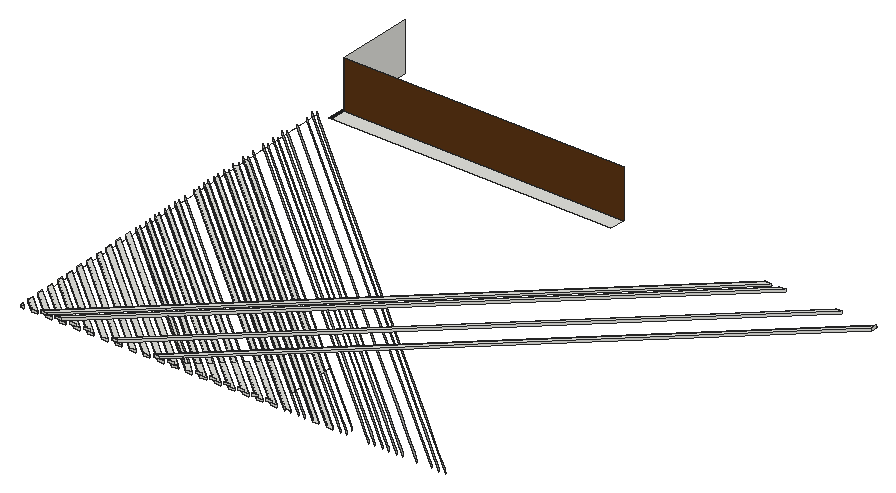
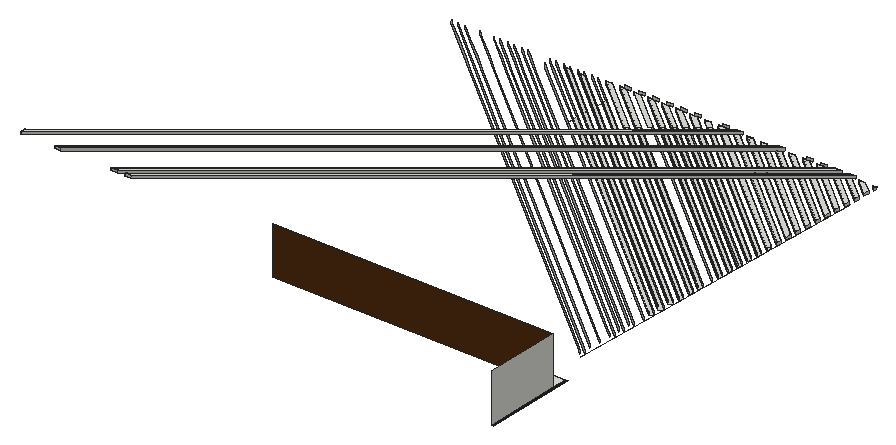
# SketchUp Ruby script. Lengths in inches.
U = 1.inch
M = Sketchup.active_model
def pt(a) = Geom::Point3d.new(a.map { |v| v * U })
def face(e, loops, mat)
  f = e.add_face(loops[0].map { |a| pt(a) })
  loops[1..].each { |l| e.add_face(l.map { |a| pt(a) }).erase! }
  f.material = f.back_material = mat if mat
  f
end
# faces: each face lists its corners as indices into pts; further lists are holes
def faces(e, pts, list, mat = nil) = list.each { |f| face(e, (f[0].is_a?(Array) ? f : [f]).map { |l| l.map { |i| pts[i] } }, mat) }
# xy, xz, yz: faces in a plane at the given z, y or x. An outline is a flat list of corners, or four numbers for a rectangle; further outlines are holes
def ring(l) = l.size == 4 ? [[l[0], l[1]], [l[2], l[1]], [l[2], l[3]], [l[0], l[3]]] : l.each_slice(2).to_a
def flat(e, list, mat, &to3) = list.each { |f| face(e, (f[0].is_a?(Array) ? f : [f]).map { |l| ring(l).map { |u, v| to3.(u, v) } }, mat) }
def xy(e, z, list, mat = nil) = flat(e, list, mat) { |x, y| [x, y, z] }
def xz(e, y, list, mat = nil) = flat(e, list, mat) { |x, z| [x, y, z] }
def yz(e, x, list, mat = nil) = flat(e, list, mat) { |y, z| [x, y, z] }
def lines(e, pts, list) = list.each { |a, b| e.add_line(pt(pts[a]), pt(pts[b])) }
# prism: a flat outline (further loops are holes) pulled along v
def prism(e, loops, v, mat = nil)
  f = face(e, loops, mat); d = Geom::Vector3d.new(v.map { |x| x * U })
  f.pushpull(f.normal.samedirection?(d) ? d.length : -d.length)
end
def box(e, o, s, mat = nil) = prism(e, [[o, [o[0] + s[0], o[1], o[2]], [o[0] + s[0], o[1] + s[1], o[2]], [o[0], o[1] + s[1], o[2]]]], [0, 0, s[2]], mat)
def at(x, y, z, deg = 0) = Geom::Transformation.translation(pt([x, y, z])) * Geom::Transformation.rotation(ORIGIN, Z_AXIS, deg.degrees)
def axes(o, x, y, z) = Geom::Transformation.new([*x, 0, *y, 0, *z, 0, *pt(o).to_a, 1])
def part(name) = M.definitions.add(name)
# library, detail: a bought-in or finely detailed component or shape, given as its bounding box
def library(name, o, s) = part(name).tap { |d| box(d.entities, o, s) }
def detail(e, o, s) = box(e.add_group.entities, o, s)
def put(e, d, t, mat = nil) = e.add_instance(d, t).tap { |i| i.material = mat if mat }
def group(e, t, mat = nil) = e.add_group.tap { |g| g.transformation = t; g.material = mat if mat }.entities
root = M.entities
M.materials.add("Wood066_2K_Color").color = [89, 51, 19]
M.materials.add("[Color M08]").color = [30, 30, 30]
xy(root,106.05,[[1644.4,661.04,1766.5625,667.76]])
xy(root,106.05,[[1643.34,661.04,1644.4,701.28]],"[Color M08]")
xz(root,667.76,[[1644.4,106.05,1766.5625,126.94]],"Wood066_2K_Color")
yz(root,1643.83,[[491.91,106.32,491.89,107.35,493.14,107.39,493.16,106.36],[496.17,106.47,498.52,106.55,498.5,107.58,496.15,107.5],[501.54,106.66,503.82,106.74,503.8,107.77,501.51,107.6875],[506.83,106.85,506.8125,107.875,509.17,107.96,509.1875,106.93],[512.2,107.04,512.18,108.06,514.47,108.15,514.49,107.12,512.95,107.0625],
  [517.5,107.23,517.48,108.25,519.83,108.34,519.85,107.31],[522.86,107.42,525.15,107.5,525.13,108.52,522.84,108.44],[528.16,107.6,530.51,107.6875,530.49,108.71,528.14,108.63],[533.53,107.79,535.74,107.87,535.72,108.9,533.5,108.82],[544.19,108.17,546.48,108.25,546.46,109.28,544.17,109.2]])
yz(root,1644.4,[[667.76,106.05,701.28,126.94]])
yz(root,1888.28,[[651.33,113.03,653.62,113.11,653.6,114.14,651.31,114.05]])
p = [[1673.29,491.89,107.35],[1643.83,517.48,108.25],[1643.83,517.5,107.23],[1673.29,491.91,106.32],[1643.83,519.85,107.31],[1676,491.91,106.32],
  [1676,491.89,107.35],[1643.83,519.83,108.34],[1643.83,512.2,107.04],[1643.83,512.95,107.0625],[1645.61,512.95,107.0625],[1669.83,491.91,106.32],
  [1667.19,491.91,106.32],[1643.83,514.49,107.12],[1643.83,514.47,108.15],[1669.83,491.89,107.35],[1667.19,491.89,107.35],[1643.83,512.18,108.06],
  [1643.83,493.16,106.36],[1645.27,491.91,106.32],[1643.83,491.91,106.32],[1645.27,491.89,107.35],[1643.83,491.89,107.35],[1643.83,493.14,107.39],
  [1643.83,496.17,106.47],[1643.83,496.15,107.5],[1648.74,491.89,107.35],[1648.74,491.91,106.32],[1643.83,498.52,106.55],[1651.45,491.91,106.32],
  [1651.45,491.89,107.35],[1643.83,498.5,107.58],[1691.74,491.91,106.32],[1643.83,533.53,107.79],[1643.83,535.74,107.87],[1643.87,535.78,107.875],
  [1694.38,491.91,106.32],[1691.74,491.89,107.35],[1643.83,533.5,108.82],[1679.47,491.91,106.32],[1643.83,522.86,107.42],[1643.83,525.15,107.5],
  [1682.1,491.91,106.32],[1679.47,491.89,107.35],[1643.83,522.84,108.44],[1682.1,491.89,107.35],[1643.83,525.13,108.52],[1697.84,491.91,106.32],
  [1643.83,538.83,107.98],[1643.83,541.18,108.07],[1700.55,491.91,106.32],[1700.55,491.89,107.35],[1643.81,541.19,108.07],[1643.81,541.17,109.09],
  [1643.83,541.16,109.09],[1697.84,491.89,107.35],[1643.83,538.8,109.01],[1710.12,491.89,107.35],[1643.83,549.47,109.39],[1643.83,549.49,108.36],
  [1710.12,491.91,106.32],[1643.83,551.84,108.44],[1712.83,491.91,106.32],[1712.83,491.89,107.35],[1643.83,551.82,109.47],[1711.88,492.72,107.375],
  [1716.3,491.91,106.32],[1643.83,554.85,108.55],[1643.83,557.14,108.63],[1718.93,491.91,106.32],[1713.61,494.22,107.43],[1643.83,554.83,109.58],
  [1716.3,491.89,107.35],[1714.93,495.37,107.47],[1718.93,491.89,107.35],[1643.83,557.12,109.66],[1722.4,491.91,106.32],[1643.83,560.15,108.74],
  [1643.83,562.51,108.82],[1725.11,491.91,106.32],[1716.66,496.87,107.52],[1643.83,560.13,109.76],[1722.4,491.89,107.35],[1718.02,498.05,107.5625],
  [1725.11,491.89,107.35],[1643.83,562.48,109.85],[1728.57,491.91,106.32],[1643.83,565.52,108.93],[1643.82,567.81,109.01],[1731.21,491.91,106.32],
  [1719.75,499.55,107.62],[1643.83,565.49,109.95],[1728.57,491.89,107.35],[1721.07,500.7,107.66],[1731.21,491.89,107.35],[1643.82,567.78,110.04],
  [1734.67,491.91,106.32],[1643.82,570.82,109.12],[1643.82,573.17,109.2],[1737.38,491.91,106.32],[1722.8,502.2,107.71],[1643.82,570.79,110.14],
  [1734.67,491.89,107.35],[1724.16,503.38,107.75],[1737.38,491.89,107.35],[1643.82,573.15,110.23],[1657.55,491.89,107.35],[1657.55,491.91,106.32],
  [1643.83,503.82,106.74],[1643.83,503.8,107.77],[1654.91,491.91,106.32],[1643.83,501.54,106.66],[1654.91,491.89,107.35],[1643.83,501.51,107.6875],
  [1740.85,491.91,106.32],[1643.82,576.18,109.31],[1643.82,578.47,109.39],[1743.49,491.92,106.32],[1725.89,504.89,107.81],[1643.82,576.16,110.33],
  [1740.85,491.89,107.35],[1727.21,506.03,107.85],[1743.49,491.89,107.35],[1643.82,578.45,110.41],[1663.72,491.89,107.35],[1663.72,491.91,106.32],
  [1643.83,509.1875,106.93],[1643.83,509.17,107.96],[1661.01,491.91,106.32],[1643.83,506.83,106.85],[1661.01,491.89,107.35],[1643.83,506.8125,107.875],
  [1753.93,501.88,106.67],[1765.4,491.92,106.32],[1765.4,491.89,107.35],[1738.16,515.55,108.18],[1643.82,597.48,111.09],[1643.82,597.51,110.0625],
  [1643.82,599.8,110.14],[1643.82,599.77,111.17],[1739.48,516.7,108.22],[1768.04,491.89,107.35],[1768.04,491.92,106.32],[1753.93,504.17,106.75],
  [1735.08,512.87,108.09],[1643.82,592.12,110.9],[1643.82,592.14,109.87],[1753.93,496.51,106.48],[1759.23,491.92,106.32],[1759.23,491.89,107.35],
  [1736.43,514.05,108.13],[1761.9375,491.89,107.35],[1761.9375,491.92,106.32],[1753.93,498.87,106.56],[1643.82,594.5,109.96],[1643.82,594.47,110.98],
  [1753.93,517.84,107.24],[1783.78,491.92,106.32],[1783.78,491.89,107.35],[1782.87,492.6875,107.375],[1781.3,494.05,107.42],[1778.04,496.88,107.52],
  [1747.35,523.53,108.47],[1643.82,613.45,111.65],[1643.82,613.47,110.63],[1728.9375,507.54,107.9],[1643.82,581.46,110.52],[1643.82,581.48,109.49],
  [1746.95,491.92,106.32],[1746.95,491.89,107.35],[1732.03,510.22,108],[1643.82,586.82,110.71],[1643.82,586.84,109.68],[1753.13,491.92,106.32],
  [1753.13,491.89,107.35],[1643.82,589.13,109.77],[1753.93,493.5,106.375],[1753.93,491.92,106.32],[1733.34,511.36,108.04],[1755.76,491.89,107.35],
  [1755.76,491.92,106.32],[1643.82,589.11,110.79],[1685.57,491.89,107.35],[1643.83,528.14,108.63],[1643.83,528.16,107.6],[1685.57,491.91,106.32],
  [1643.83,530.51,107.6875],[1688.28,491.91,106.32],[1688.28,491.89,107.35],[1643.83,530.49,108.71],[1753.93,507.18,106.86],[1643.82,602.81,110.25],
  [1645.18,603.98,110.29],[1774.21,491.92,106.32],[1771.5,491.92,106.32],[1771.5,491.89,107.35],[1741.21,518.2,108.28],[1643.82,602.78,111.28],
  [1753.93,512.54,107.05],[1753.93,512.95,107.0625],[1753.46,512.95,107.0625],[1643.82,608.17,110.44],[1645.14,609.32,110.48],[1780.32,491.92,106.32],
  [1777.68,491.92,106.32],[1777.68,491.89,107.35],[1774.99,494.23,107.43],[1744.3,520.88,108.375],[1643.82,608.15,111.47],[1704.02,491.91,106.32],
  [1643.83,544.19,108.17],[1643.83,546.48,108.25],[1706.66,491.91,106.32],[1643.83,546.46,109.28],[1706.66,491.89,107.35],[1704.02,491.89,107.35],
  [1643.83,544.17,109.2],[1753.93,528.5,107.62],[1796.06,491.92,106.32],[1796.06,491.9,107.35],[1792.05,495.375,107.47],[1784.18,502.22,107.71],
  [1753.49,528.87,108.66],[1643.82,624.11,112.03],[1643.82,624.13,111.01],[1753.93,533.87,107.81],[1802.23,491.92,106.32],[1802.23,491.9,107.35],
  [1795.14,498.06,107.5625],[1787.26,504.9,107.81],[1756.58,531.55,108.75],[1643.82,629.48,112.22],[1643.82,629.5,111.2],[1753.93,539.17,107.99],
  [1808.33,491.92,106.32],[1808.33,491.9,107.35],[1798.19,500.71,107.66],[1790.3125,507.55,107.9],[1759.625,534.2,108.85],[1643.82,634.77,112.41],
  [1643.82,634.8,111.38],[1753.93,555.2,108.5625],[1826.79,491.92,106.32],[1826.79,491.9,107.35],[1817.97,499.56,107.62],[1807.42,508.72,107.94],
  [1799.54,515.5625,108.18],[1768.85,542.21,109.13],[1647.16,647.9,112.875],[1643.82,650.8,112.98],[1643.82,650.82,111.95],[1694.38,491.89,107.35],
  [1643.87,535.76,108.9],[1776.3,495.38,107.47],[1780.32,491.89,107.35],[1645.14,609.29,111.51],[1645.82,608.7,111.49],[1745.62,522.03,108.41],
  [1797.77,498.06,107.5625],[1803.55,493.04,107.39],[1803.91,492.73,107.375],[1804.87,491.9,107.35],[1804.87,491.92,106.32],[1753.93,536.16,107.89],
  [1648.23,627.96,111.14],[1645.14,630.64,111.24],[1645.14,630.62,112.26],[1645.85,630,112.24],[1757.89,532.69,108.79],[1788.58,506.04,107.85],
  [1796.46,499.2,107.6],[1813.15,495.37,107.47],[1815.83,493.04,107.39],[1817.15,491.9,107.35],[1817.15,491.92,106.32],[1753.93,546.82,108.27],
  [1645.14,641.31,111.61],[1645.14,641.28,112.64],[1645.91,640.62,112.62],[1648.65,638.24,112.53],[1764.03,538.02,108.98],[1794.72,511.375,108.04],
  [1802.6,504.53,107.79],[1812.16,496.23,107.5],[1819.29,500.7,107.66],[1828.1,493.04,107.39],[1829.42,491.9,107.35],[1829.42,491.92,106.32],
  [1753.93,557.48,108.64],[1649.02,648.59,111.875],[1645.14,651.97,111.99],[1645.14,651.95,113.02],[1648.69,648.86,112.91],[1770.17,543.36,109.17],
  [1800.86,516.71,108.23],[1808.73,509.86,107.98],[1783.12,494.82,107.45],[1784.22,493.86,107.42],[1786.49,491.9,107.35],[1786.49,491.92,106.32],
  [1781.35,496.38,106.48],[1753.93,520.19,107.32],[1645.18,614.65,110.67],[1645.18,614.625,111.7],[1645.43,614.4,111.6875],[1748.71,524.71,108.51],
  [1779.39,498.06,107.5625],[1773.25,492.73,107.375],[1774.21,491.89,107.35],[1645.18,603.96,111.32],[1645.47,603.71,111.31],[1742.57,519.38,108.32],
  [1811.04,491.9,107.35],[1811.04,491.92,106.32],[1753.93,541.52,108.08],[1649.32,632.37,111.3],[1645.17,635.97,111.43],[1645.17,635.95,112.45],
  [1648.86,632.75,112.34],[1760.98,535.375,108.89],[1791.67,508.72,107.94],[1799.55,501.88,107.7],[1807.24,495.2,107.46],[1810.1,492.72,107.375],
  [1793.41,496.55,107.51],[1797.41,493.07,107.39],[1798.77,491.9,107.35],[1798.77,491.92,106.32],[1753.93,530.86,107.7],[1645.17,625.31,111.05],
  [1645.17,625.29,112.07],[1648.82,622.12,111.96],[1754.84,530.04,108.7],[1785.53,503.39,107.75],[1788.05,501.21,107.68],[1797.81,514.06,108.13],
  [1802.64,509.86,107.98],[1805.68,507.21,107.89],[1816.24,498.05,107.5625],[1823.32,491.9,107.35],[1823.32,491.92,106.32],[1753.93,552.18,108.46],
  [1649.5,642.88,111.67],[1645.17,646.64,111.8],[1645.17,646.61,112.83],[1648.5,643.72,112.73],[1767.12,540.71,109.08],[1655.64,491.89,107.35],
  [1661.81,491.89,107.35],[1667.91,491.89,107.35],[1674.09,491.89,107.35],[1686.36,491.89,107.35],[1704.74,491.89,107.35],[1712.46,491.89,107.35],
  [1710.93,491.89,107.35],[1723.19,491.89,107.35],[1729.3,491.89,107.35],[1735.47,491.89,107.35],[1741.57,491.89,107.35],[1749.66,491.89,107.35],
  [1749.66,491.92,106.32],[1747.75,491.89,107.35],[1753.85,491.89,107.35],[1784.75,496.44,106.48],[1785.96,495.39,106.44],[1785.96,495.37,107.47],
  [1782.86,498.06,107.5625],[1781.125,499.57,107.62],[1750.4375,526.22,108.5625],[1643.82,618.8125,111.85],[1643.82,618.83,110.82],[1753.93,523.21,107.43],
  [1643.83,535.72,108.9],[1653,491.89,107.375],[1653,491.89,107.35],[1655.64,491.89,107.375],[1655.64,491.86,108.4],[1653,491.86,108.4],
  [1659.1,491.86,108.4],[1659.1,491.89,107.375],[1659.1,491.89,107.35],[1661.81,491.89,107.375],[1661.81,491.86,108.4],[1665.28,491.89,107.35],
  [1667.91,491.89,107.375],[1667.91,491.86,108.4],[1665.28,491.86,108.4],[1665.28,491.89,107.375],[1671.38,491.89,107.35],[1674.09,491.89,107.375],
  [1674.09,491.87,108.4],[1671.38,491.86,108.4],[1671.38,491.89,107.375],[1683.65,491.89,107.375],[1683.65,491.89,107.35],[1686.36,491.89,107.375],
  [1686.36,491.87,108.4],[1683.65,491.87,108.4],[1702.11,491.87,108.4],[1702.11,491.89,107.375],[1702.11,491.89,107.35],[1704.74,491.89,107.375],
  [1704.74,491.87,108.4],[1708.21,491.87,108.4],[1708.21,491.89,107.375],[1708.21,491.89,107.35],[1710.93,491.87,108.4],[1710.92,491.87,108.4],
  [1723.19,491.87,108.4],[1723.19,491.89,107.375],[1720.48,491.89,107.35],[1720.48,491.89,107.375],[1720.48,491.87,108.4],[1726.66,491.89,107.35],
  [1726.66,491.89,107.375],[1726.66,491.87,108.4],[1729.3,491.87,108.4],[1729.3,491.89,107.375],[1730.29,508.71,107.94],[1732.76,491.89,107.35],
  [1732.76,491.89,107.375],[1732.76,491.87,108.4],[1735.47,491.87,108.4],[1735.47,491.89,107.375],[1760.02,491.89,107.35],[1738.9375,491.89,107.375],
  [1738.9375,491.87,108.4],[1741.57,491.87,108.4],[1741.57,491.89,107.375],[1738.9375,491.89,107.35],[1745.04,491.89,107.35],[1745.04,491.89,107.375],
  [1745.04,491.87,108.4],[1747.75,491.87,108.4],[1747.75,491.89,107.375],[1751.21,491.89,107.375],[1751.21,491.87,108.4],[1753.85,491.87,108.4],
  [1753.85,491.89,107.375],[1751.21,491.89,107.35],[1839.55,653.94,113.12],[1839.55,653.92,114.15],[1842.18,653.92,114.15],[1842.18,653.94,113.12],
  [1845.65,653.94,113.12],[1845.65,653.92,114.15],[1848.36,653.92,114.15],[1848.36,653.94,113.12],[1870.2,653.94,113.12],[1870.2,653.92,114.15],
  [1872.91,653.92,114.15],[1872.91,653.94,113.12],[1888.28,653.62,113.11],[1888.28,653.6,114.14],[1888.28,651.31,114.05],[1888.28,651.33,113.03],
  [1643.83,535.82,107.875],[1661.45,603.7,106.47],[1661.42,603.7,106.47],[1644.33,653.02,111.26],[1643.93,505.92,106.4375]]
faces(root,p,[[0,1,2,3],[3,2,4,5],[6,5,4,7],[8,9,10,11,12],[10,13,14,15,11],[16,17,8,12],[18,19,20],[21,22,20,19],
  [19,18,23,21],[24,25,26,27],[28,29,27,24],[30,29,28,31],[32,33,34,35,36],[37,38,33,32],[39,40,41,42],[43,44,40,39],
  [45,42,41,46],[47,48,49,50],[51,50,49,52,53,54],[55,56,48,47],[57,58,59,60],[60,59,61,62],[63,62,61,64,65],[66,67,68,69],
  [70,71,67,66,72],[73,74,69,68,75],[76,77,78,79],[80,81,77,76,82],[83,84,79,78,85],[86,87,88,89],[90,91,87,86,92],[93,94,89,88,95],
  [96,97,98,99],[100,101,97,96,102],[103,104,99,98,105],[106,107,108,109],[108,107,110,111],[112,113,111,110],[114,115,116,117],[118,119,115,114,120],
  [121,122,117,116,123],[124,125,126,127],[126,125,128,129],[130,131,129,128],[132,133,134,135,136,137],[138,139,140,141,142,143],[144,145,146,147,148,149],[150,151,152,153,154,155],
  [156,157,158,159,160,161,162,163,164],[165,166,167,168,169],[170,171,172,173,174],[173,172,175,176,177],[178,179,180,176,175,181],[182,183,184,185],[185,184,186,187],[188,187,186,189],
  [190,191,192,193,194],[190,194,195,196,197,191],[198,199,200,201,202,203,204],[198,204,205,206,207,208,201,200],[209,210,211,212],[212,211,213,214],[215,216,210,209],[217,218,219,220,221,222,223,224],
  [225,226,227,228,229,230,231,232],[233,234,235,236,237,238,239,240],[241,242,243,244,245,246,247,248,249,250],[251,36,35,252],[253,254,203,202,255,256,257],[258,259,260,261,262,263,264,265,266,267,268,269,270],[271,272,273,274,275,276,277,278,279,280,281,282,283],[284,285,286,287,288,289,290,291,292,293,294,295],
  [296,297,298,299,300,301,302,303,304,305,306],[307,308,193,192,309,310,311],[312,313,314,315,316,317,318,319,320,321,322,323],[324,325,326,327,328,329,330,331,332,333,334],[335,336,337,338,339,340,341,342,343,344,345,346],[26,27,29,30],[347,112,110,107,106],[124,348,130,128,125],
  [11,15,349,16,12],[6,350,0,3,5],[42,45,43,39],[351,182,185,187,188],[251,37,32,36],[51,55,47,50],[212,214,352,215,209],[62,63,353,354,57,60],
  [72,66,69,74],[82,355,84,79,76],[86,92,356,94,89],[102,357,104,99,96],[114,120,358,122,117],[359,360,168,169,361],[173,174,362,179,180,177],[176,180,177],
  [363,364,365,366,367,368,369,370,371],[147,146,154,153],[132,137,138,143],[198,200,199],[13,10,9],[302,301,156,164],[6,7,1,0,350],[15,14,17,16,349],
  [22,21,23],[30,31,25,26],[252,372,38,37,251],[45,46,44,43],[51,54,56,55],[65,64,58,57,354],[106,109,113,112,347],[124,127,131,130,348],
  [188,189,183,182,351],[214,213,216,215,352],[373,374,112,347,375,376,377],[378,379,380,130,348,381,382],[383,16,349,384,385,386,387],[388,0,350,389,390,391,392],[393,394,182,351,395,396,397],[398,399,400,215,352,401,402],
  [403,404,405,57,354,406,407],[63,65,354,353],[70,72,74,73],[80,82,355,84,83],[90,92,356,94,93],[408,409,355,82,410,411,412],[100,102,357,104,103],[118,120,358,122,121],
  [413,414,415,416,417,356,92],[359,418,165,169,361],[179,178,170,174,362],[419,420,421,422,423,357,102],[151,150,144,149,424],[425,426,427,428,358,120,429],[169,430,431,432,433,434,361],[435,436,437,438,362,174,439],
  [440,373,377,441],[442,376,375,443],[444,379,378,445],[446,382,381,447],[448,393,397,449],[450,396,395,451],[452,399,398,453],[454,402,401,455],
  [35,34,372,252],[35,34,456],[49,48,52],[52,53,56,48],[441,377,376,442],[445,378,382,446],[449,397,396,450],[453,398,402,454],
  [54,53,56],[441,442,443,440],[445,446,447,444],[449,450,451,448]])
lines(root,p,[[457,458],[190,143],[371,301],[459,460]])
